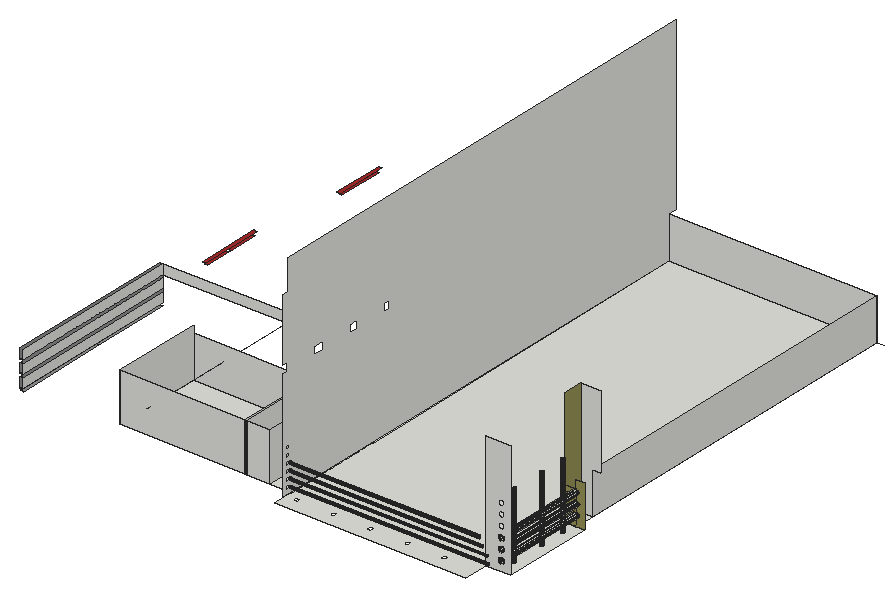
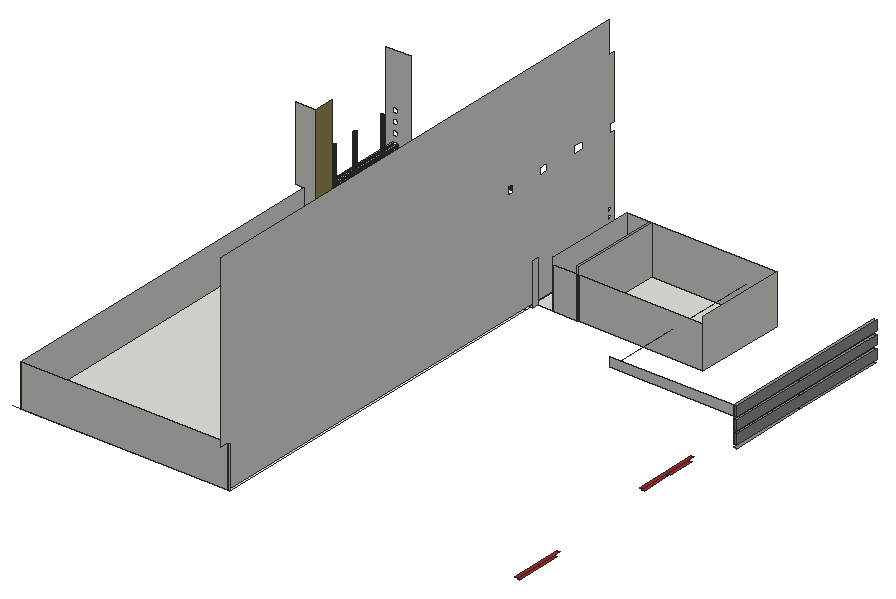
# SketchUp Ruby script. Lengths in inches.
U = 1.inch
M = Sketchup.active_model
def pt(a) = Geom::Point3d.new(a.map { |v| v * U })
def face(e, loops, mat)
  f = e.add_face(loops[0].map { |a| pt(a) })
  loops[1..].each { |l| e.add_face(l.map { |a| pt(a) }).erase! }
  f.material = f.back_material = mat if mat
  f
end
# faces: each face lists its corners as indices into pts; further lists are holes
def faces(e, pts, list, mat = nil) = list.each { |f| face(e, (f[0].is_a?(Array) ? f : [f]).map { |l| l.map { |i| pts[i] } }, mat) }
# xy, xz, yz: faces in a plane at the given z, y or x. An outline is a flat list of corners, or four numbers for a rectangle; further outlines are holes
def ring(l) = l.size == 4 ? [[l[0], l[1]], [l[2], l[1]], [l[2], l[3]], [l[0], l[3]]] : l.each_slice(2).to_a
def flat(e, list, mat, &to3) = list.each { |f| face(e, (f[0].is_a?(Array) ? f : [f]).map { |l| ring(l).map { |u, v| to3.(u, v) } }, mat) }
def xy(e, z, list, mat = nil) = flat(e, list, mat) { |x, y| [x, y, z] }
def xz(e, y, list, mat = nil) = flat(e, list, mat) { |x, z| [x, y, z] }
def yz(e, x, list, mat = nil) = flat(e, list, mat) { |y, z| [x, y, z] }
def lines(e, pts, list) = list.each { |a, b| e.add_line(pt(pts[a]), pt(pts[b])) }
# prism: a flat outline (further loops are holes) pulled along v
def prism(e, loops, v, mat = nil)
  f = face(e, loops, mat); d = Geom::Vector3d.new(v.map { |x| x * U })
  f.pushpull(f.normal.samedirection?(d) ? d.length : -d.length)
end
def box(e, o, s, mat = nil) = prism(e, [[o, [o[0] + s[0], o[1], o[2]], [o[0] + s[0], o[1] + s[1], o[2]], [o[0], o[1] + s[1], o[2]]]], [0, 0, s[2]], mat)
def at(x, y, z, deg = 0) = Geom::Transformation.translation(pt([x, y, z])) * Geom::Transformation.rotation(ORIGIN, Z_AXIS, deg.degrees)
def axes(o, x, y, z) = Geom::Transformation.new([*x, 0, *y, 0, *z, 0, *pt(o).to_a, 1])
def part(name) = M.definitions.add(name)
# library, detail: a bought-in or finely detailed component or shape, given as its bounding box
def library(name, o, s) = part(name).tap { |d| box(d.entities, o, s) }
def detail(e, o, s) = box(e.add_group.entities, o, s)
def put(e, d, t, mat = nil) = e.add_instance(d, t).tap { |i| i.material = mat if mat }
def group(e, t, mat = nil) = e.add_group.tap { |g| g.transformation = t; g.material = mat if mat }.entities
root = M.entities
M.materials.add("[0018_Brown]").color = [165, 42, 42]
M.materials.add("[0057_DarkKhaki]").color = [150, 145, 85]
M.materials.add("[0137_Black]").color = [71, 71, 71]
M.materials.add("[Color M05]").color = [145, 145, 145]
xy(root,378.28,[[8.875,19,11.875,116.75],[8.875,116.75,11.875,199.5]],"[Color M05]")
xy(root,379.4,[[8.875,431.78,11.875,479.72]],"[0018_Brown]")
xy(root,379.43,[[[286.99,1.0625,484.5625,1.0625,484.5625,26.4375,510.6875,26.4375,510.6875,122.75,490.125,122.75,490.125,143.77,501.6875,143.77,501.6875,511.875,286.99,511.875],[412.39,12.9375,411.69,13.03,411.04,13.3,410.49,13.73,410.06,14.28,409.79,14.93,409.7,15.625,409.79,16.32,410.06,16.97,410.49,17.53,411.04,17.95,411.69,18.22,412.39,18.3125,413.08,18.22,413.73,17.95,414.29,17.53,414.72,16.97,414.98,16.32,415.07,15.625,414.98,14.93,414.71,14.28,414.29,13.72,413.73,13.3,413.08,13.03],[450.64,12.9375,449.94,13.03,449.29,13.3,448.74,13.73,448.31,14.28,448.04,14.93,447.95,15.625,448.04,16.32,448.31,16.97,448.74,17.53,449.29,17.95,449.94,18.22,450.64,18.3125,451.33,18.22,451.98,17.95,452.54,17.53,452.97,16.97,453.23,16.32,453.32,15.625,453.23,14.93,452.96,14.28,452.54,13.72,451.98,13.3,451.33,13.03],[297.64,12.9375,296.94,13.03,296.29,13.3,295.74,13.73,295.31,14.28,295.04,14.93,294.95,15.625,295.04,16.32,295.31,16.97,295.74,17.53,296.29,17.95,296.94,18.22,297.64,18.3125,298.33,18.22,298.98,17.95,299.54,17.53,299.97,16.97,300.23,16.32,300.32,15.625,300.23,14.93,299.96,14.28,299.54,13.72,298.98,13.3,298.33,13.03],[335.89,12.9375,335.19,13.03,334.54,13.3,333.99,13.73,333.56,14.28,333.29,14.93,333.2,15.625,333.29,16.32,333.56,16.97,333.99,17.53,334.54,17.95,335.19,18.22,335.89,18.3125,336.58,18.22,337.23,17.95,337.79,17.53,338.22,16.97,338.48,16.32,338.57,15.625,338.48,14.93,338.21,14.28,337.79,13.72,337.23,13.3,336.58,13.03],[374.14,12.9375,373.44,13.03,372.79,13.3,372.24,13.73,371.81,14.28,371.54,14.93,371.45,15.625,371.54,16.32,371.81,16.97,372.24,17.53,372.79,17.95,373.44,18.22,374.14,18.3125,374.83,18.22,375.48,17.95,376.04,17.53,376.47,16.97,376.73,16.32,376.82,15.625,376.73,14.93,376.46,14.28,376.04,13.72,375.48,13.3,374.83,13.03],[499.41,79.41,499.04,79.46,498.6875,79.61,498.39,79.84,498.16,80.13,498.02,80.48,497.97,80.85,498.02,81.22,498.16,81.57,498.39,81.87,498.6875,82.1,499.04,82.24,499.41,82.29,499.78,82.24,500.125,82.1,500.42,81.87,500.65,81.57,500.8,81.22,500.85,80.85,500.8,80.48,500.65,80.13,500.42,79.84,500.125,79.61,499.78,79.46],[499.41,107.04,499.04,107.09,498.6875,107.23,498.39,107.46,498.16,107.76,498.02,108.11,497.97,108.48,498.02,108.85,498.16,109.2,498.39,109.49,498.6875,109.72,499.04,109.87,499.41,109.91,499.78,109.87,500.125,109.72,500.42,109.49,500.65,109.2,500.8,108.85,500.85,108.48,500.8,108.11,500.65,107.76,500.42,107.46,500.125,107.23,499.78,107.09],[499.41,44.29,499.04,44.34,498.6875,44.48,498.39,44.71,498.16,45.01,498.02,45.36,497.97,45.73,498.02,46.1,498.16,46.45,498.39,46.74,498.6875,46.97,499.04,47.12,499.41,47.16,499.78,47.12,500.125,46.97,500.42,46.74,500.65,46.45,500.8,46.1,500.85,45.73,500.8,45.36,500.65,45.01,500.42,44.71,500.125,44.48,499.78,44.34]],[286.17,18.1875,286.99,22.0625],[284.05,22.0625,284.05,22.07,284.41,22.0625],[284.41,22.0625,284.05,22.07,284.05,116.75,284.41,116.75],[284.41,22.0625,284.41,116.75,285.29,116.75],
  [284.41,22.0625,285.29,116.75,285.29,22.0625],[285.29,22.0625,286.17,116.75],[286.17,22.0625,286.99,116.75],[284.05,22.07,264.04,22.25,264.92,116.9375,281.04,116.79,281.04,116.75,284.05,116.75],[264.04,22.25,239.85,22.47,240.73,117.16,264.92,116.9375],
  [239.85,22.47,237.79,22.49,238.67,117.18,240.73,117.16],[237.79,22.49,107.8,23.69,108.67,118.38,238.67,117.18],[281.04,116.75,281.04,116.79,284.05,116.76,284.05,116.75],[284.05,116.75,284.05,116.76,285.29,116.75],[285.29,116.75,284.05,116.76,284.05,122.75,285.29,122.75],
  [285.29,116.75,286.17,122.75],[286.17,116.75,286.99,122.75],[284.05,116.76,281.04,116.79,281.04,122.75,284.05,122.75],[284.05,122.75,286.17,128.75],[286.17,122.75,286.99,128.75],
  [490.125,122.75,501.6875,143.77],[284.05,128.75,286.17,511.875],[286.17,128.75,286.99,511.875]])
xy(root,381.32,[[8.875,18.1875,11.875,199.5]])
xy(root,382.4,[[8.875,428.78,11.875,482.72]],"[0018_Brown]")
xy(root,391.28,[[8.875,257.47,11.875,284.61],[8.875,287.91,11.875,318.35]],"[0018_Brown]")
xy(root,391.4,[[8.875,18.1875,11.875,116.75],[8.875,116.75,11.875,199.5]],"[Color M05]")
xy(root,394.28,[[8.875,254.47,11.875,321.35]],"[0018_Brown]")
xy(root,394.44,[[8.875,18.1875,11.875,199.5]])
xy(root,404.53,[[8.875,18.1875,11.875,116.75],[8.875,116.75,11.875,199.5]],"[Color M05]")
xy(root,407.57,[[8.875,18.1875,11.875,199.5]])
xz(root,26.4375,[[[484.5625,379.43,510.6875,499.43],[501.3,386.68,502.06,386.78,502.77,387.07,503.375,387.54,503.84,388.15,504.13,388.85,504.23,389.62,504.13,390.375,503.84,391.08,503.375,391.69,502.77,392.16,502.06,392.45,501.3,392.55,500.54,392.45,499.83,392.16,499.22,391.69,498.75,391.08,498.46,390.375,498.36,389.62,498.46,388.85,498.75,388.15,499.22,387.54,499.83,387.07,500.54,386.78],[501.3,397.43,502.06,397.53,502.77,397.82,503.375,398.29,503.84,398.9,504.13,399.6,504.23,400.37,504.13,401.125,503.84,401.83,503.375,402.44,502.77,402.91,502.06,403.2,501.3,403.3,500.54,403.2,499.83,402.91,499.22,402.44,498.75,401.83,498.46,401.125,498.36,400.37,498.46,399.6,498.75,398.9,499.22,398.29,499.83,397.82,500.54,397.53],[501.3,408.18,502.06,408.28,502.77,408.57,503.375,409.04,503.84,409.65,504.13,410.35,504.23,411.12,504.13,411.875,503.84,412.58,503.375,413.19,502.77,413.66,502.06,413.95,501.3,414.05,500.54,413.95,499.83,413.66,499.22,413.19,498.75,412.58,498.46,411.875,498.36,411.12,498.46,410.35,498.75,409.65,499.22,409.04,499.83,408.57,500.54,408.28],[501.3,418.93,502.06,419.03,502.77,419.32,503.375,419.79,503.84,420.4,504.13,421.1,504.23,421.87,504.13,422.625,503.84,423.33,503.375,423.94,502.77,424.41,502.06,424.7,501.3,424.8,500.54,424.7,499.83,424.41,499.22,423.94,498.75,423.33,498.46,422.625,498.36,421.87,498.46,421.1,498.75,420.4,499.22,419.79,499.83,419.32,500.54,419.03],[501.3,429.68,502.06,429.78,502.77,430.07,503.375,430.54,503.84,431.15,504.13,431.85,504.23,432.62,504.13,433.375,503.84,434.08,503.375,434.69,502.77,435.16,502.06,435.45,501.3,435.55,500.54,435.45,499.83,435.16,499.22,434.69,498.75,434.08,498.46,433.375,498.36,432.62,498.46,431.85,498.75,431.15,499.22,430.54,499.83,430.07,500.54,429.78],[501.3,440.43,502.06,440.53,502.77,440.82,503.375,441.29,503.84,441.9,504.13,442.6,504.23,443.37,504.13,444.125,503.84,444.83,503.375,445.44,502.77,445.91,502.06,446.2,501.3,446.3,500.54,446.2,499.83,445.91,499.22,445.44,498.75,444.83,498.46,444.125,498.36,443.37,498.46,442.6,498.75,441.9,499.22,441.29,499.83,440.82,500.54,440.53]]])
xz(root,122.75,[[501.3,408.18,500.91,408.23,501.6875,408.23],[500.91,408.23,500.54,408.28,499.83,408.57,499.22,409.04,498.75,409.65,498.46,410.35,498.36,411.12,498.46,411.875,498.75,412.58,499.22,413.19,499.83,413.66,500.54,413.95,500.91,414,501.6875,414,501.6875,408.23],[501.6875,408.23,501.6875,414,502.06,413.95,502.77,413.66,503.375,413.19,503.84,412.58,504.13,411.875,504.23,411.12,504.13,410.35,503.84,409.65,503.375,409.04,502.77,408.57,502.06,408.28]])
xz(root,122.75,[[490.125,379.43,501.6875,379.43,501.6875,408.23,501.3,408.18,500.91,408.23,490.125,408.23],[501.6875,379.43,510.6875,379.43,510.6875,423,501.6875,423,501.6875,414,502.06,413.95,502.77,413.66,503.375,413.19,503.84,412.58,504.13,411.875,504.23,411.12,504.13,410.35,503.84,409.65,503.375,409.04,502.77,408.57,502.06,408.28,501.6875,408.23],[490.125,408.23,500.91,408.23,500.54,408.28,499.83,408.57,499.22,409.04,498.75,409.65,498.46,410.35,498.36,411.12,498.46,411.875,498.75,412.58,499.22,413.19,499.83,413.66,500.54,413.95,500.91,414,490.125,414]],"[0057_DarkKhaki]")
xz(root,123.3125,[[501.3,386.68,500.54,386.78,499.83,387.07,499.22,387.54,498.75,388.15,498.46,388.85,498.36,389.62,498.46,390.375,498.75,391.08,499.22,391.69,499.83,392.16,500.54,392.45,501.3,392.55,502.06,392.45,502.77,392.16,503.375,391.69,503.84,391.08,504.13,390.375,504.23,389.62,504.13,388.85,503.84,388.15,503.375,387.54,502.77,387.07,502.06,386.78]])
xz(root,127.4375,[[501.3,397.43,500.54,397.53,499.83,397.82,499.22,398.29,498.75,398.9,498.46,399.6,498.36,400.37,498.46,401.125,498.75,401.83,499.22,402.44,499.83,402.91,500.54,403.2,501.3,403.3,502.06,403.2,502.77,402.91,503.375,402.44,503.84,401.83,504.13,401.125,504.23,400.37,504.13,399.6,503.84,398.9,503.375,398.29,502.77,397.82,502.06,397.53]])
xz(root,143.77,[[490.125,379.43,490.125,499.43,510.6875,499.43,510.6875,423,501.6875,423,501.6875,379.43]])
xz(root,199.5,[[11.875,407.57,139.9375,417.65]])
xz(root,199.5,[[8.875,381.32,11.875,391.4],[8.875,394.44,11.875,404.53],[8.875,407.57,11.875,417.65]],"[Color M05]")
xz(root,511.875,[[284.05,379.43,286.17,423],[286.17,379.43,501.6875,423]])
yz(root,8.875,[[18.1875,381.32,199.5,391.4],[18.1875,394.44,199.5,404.53],[18.1875,407.57,199.5,417.65]],"[Color M05]")
yz(root,11.875,[[19,381.32,199.5,381.32,199.5,391.4,18.1875,391.4,18.1875,381.65,19,381.65],[18.1875,394.44,199.5,404.53],[18.1875,407.57,199.5,417.65]])
yz(root,11.875,[[18.1875,391.4,199.5,394.44],[18.1875,404.53,199.5,407.57]],"[Color M05]")
yz(root,281.04,[[116.75,379.43,122.75,423]])
yz(root,286.17,[[[12.1875,379.43,511.875,379.43,511.875,423,520.875,423,520.875,599.125,18.1875,599.125,18.1875,567.22,12.1875,567.22,12.1875,501.97,16.9375,501.97,16.9375,493.97,12.1875,493.97],[51.75,493.97,63.75,501.97],[98.5625,493.97,108.4375,501.97],[143.25,493.97,149.48,501.97],[18.04,383.86,17.46,383.94,16.92,384.16,16.45,384.52,16.1,384.99,15.87,385.53,15.79,386.11,15.87,386.7,16.1,387.24,16.45,387.7,16.92,388.0625,17.46,388.29,18.04,388.36,18.63,388.29,19.17,388.0625,19.64,387.7,19.99,387.24,20.22,386.7,20.29,386.11,20.22,385.53,19.99,384.99,19.64,384.52,19.17,384.16,18.63,383.94],[18.04,391.36,17.46,391.44,16.92,391.66,16.45,392.02,16.1,392.49,15.87,393.03,15.79,393.61,15.87,394.2,16.1,394.74,16.45,395.2,16.92,395.5625,17.46,395.79,18.04,395.86,18.63,395.79,19.17,395.5625,19.64,395.2,19.99,394.74,20.22,394.2,20.29,393.61,20.22,393.03,19.99,392.49,19.64,392.02,19.17,391.66,18.63,391.44],[18.04,398.86,17.46,398.94,16.92,399.16,16.45,399.52,16.1,399.99,15.87,400.53,15.79,401.11,15.87,401.7,16.1,402.24,16.45,402.7,16.92,403.0625,17.46,403.29,18.04,403.36,18.63,403.29,19.17,403.0625,19.64,402.7,19.99,402.24,20.22,401.7,20.29,401.11,20.22,400.53,19.99,399.99,19.64,399.52,19.17,399.16,18.63,398.94],[18.04,406.36,17.46,406.44,16.92,406.66,16.45,407.02,16.1,407.49,15.87,408.03,15.79,408.61,15.87,409.2,16.1,409.74,16.45,410.2,16.92,410.5625,17.46,410.79,18.04,410.86,18.63,410.79,19.17,410.5625,19.64,410.2,19.99,409.74,20.22,409.2,20.29,408.61,20.22,408.03,19.99,407.49,19.64,407.02,19.17,406.66,18.63,406.44],[18.04,413.86,17.46,413.94,16.92,414.16,16.45,414.52,16.1,414.99,15.87,415.53,15.79,416.11,15.87,416.7,16.1,417.24,16.45,417.7,16.92,418.0625,17.46,418.29,18.04,418.36,18.63,418.29,19.17,418.0625,19.64,417.7,19.99,417.24,20.22,416.7,20.29,416.11,20.22,415.53,19.99,414.99,19.64,414.52,19.17,414.16,18.63,413.94],[18.04,421.36,17.46,421.44,16.92,421.66,16.45,422.02,16.1,422.49,15.87,423.03,15.79,423.61,15.87,424.2,16.1,424.74,16.45,425.2,16.92,425.5625,17.46,425.79,18.04,425.86,18.63,425.79,19.17,425.5625,19.64,425.2,19.99,424.74,20.22,424.2,20.29,423.61,20.22,423.03,19.99,422.49,19.64,422.02,19.17,421.66,18.63,421.44]]])
yz(root,490.125,[[122.75,379.43,143.77,499.43]],"[0057_DarkKhaki]")
yz(root,501.6875,[[143.77,379.43,511.875,423]])
p = [[264.04,22.25,429.99],[239.85,22.47,429.99],[239.85,22.47,379.43],[264.04,22.25,379.43],[264.91,116.51,429.99],[264.91,116.75,429.99],
  [264.92,116.9375,429.99],[264.92,116.9375,423],[264.92,116.9375,379.43],[107.8,23.69,379.43],[237.79,22.49,379.43],[237.79,22.49,429.99],
  [107.8,23.69,429.99],[238.66,116.75,429.99],[238.67,117.18,429.99],[238.67,117.18,423],[238.67,117.18,379.43],[240.73,116.73,429.99],
  [240.73,116.75,429.99],[240.73,117.16,429.99],[240.73,117.16,423],[240.73,117.16,379.43],[108.66,116.75,429.99],[108.67,118.38,429.99],
  [108.67,118.38,423],[108.67,118.38,379.43],[498.6875,44.48,379.43],[499.04,44.34,379.43],[499.04,44.34,448.18],[498.6875,44.48,448.18],
  [499.41,44.29,379.43],[499.41,44.29,448.18],[499.78,44.34,379.43],[499.78,44.34,448.18],[500.125,44.48,379.43],[500.125,44.48,448.18],
  [498.39,44.71,379.43],[498.39,44.71,448.18],[500.42,44.71,379.43],[500.42,44.71,448.18],[498.16,45.01,379.43],[498.16,45.01,448.18],
  [500.65,45.01,379.43],[500.65,45.01,448.18],[498.02,45.36,379.43],[498.02,45.36,448.18],[500.8,45.36,379.43],[500.8,45.36,448.18],
  [497.97,45.73,379.43],[497.97,45.73,448.18],[500.85,45.73,379.43],[500.85,45.73,448.18],[498.02,46.1,379.43],[498.02,46.1,448.18],
  [500.8,46.1,379.43],[500.8,46.1,448.18],[498.16,46.45,379.43],[498.16,46.45,448.18],[500.65,46.45,379.43],[500.65,46.45,448.18],
  [498.39,46.74,379.43],[498.39,46.74,448.18],[500.42,46.74,379.43],[500.42,46.74,448.18],[498.6875,46.97,379.43],[498.6875,46.97,448.18],
  [500.125,46.97,379.43],[500.125,46.97,448.18],[499.04,47.12,379.43],[499.04,47.12,448.18],[499.78,47.12,379.43],[499.78,47.12,448.18],
  [499.41,47.16,379.43],[499.41,47.16,448.18],[499.04,79.46,379.43],[499.41,79.41,379.43],[499.41,79.41,448.18],[499.04,79.46,448.18],
  [499.78,79.46,379.43],[499.78,79.46,448.18],[498.6875,79.61,379.43],[498.6875,79.61,448.18],[500.125,79.61,379.43],[500.125,79.61,448.18],
  [498.39,79.84,379.43],[498.39,79.84,448.18],[500.42,79.84,379.43],[500.42,79.84,448.18],[498.16,80.13,379.43],[498.16,80.13,448.18],
  [500.65,80.13,379.43],[500.65,80.13,448.18],[498.02,80.48,379.43],[498.02,80.48,448.18],[500.8,80.48,379.43],[500.8,80.48,448.18],
  [497.97,80.85,379.43],[497.97,80.85,448.18],[500.85,80.85,379.43],[500.85,80.85,448.18],[498.02,81.22,379.43],[498.02,81.22,448.18],
  [500.8,81.22,379.43],[500.8,81.22,448.18],[498.16,81.57,379.43],[498.16,81.57,448.18],[500.65,81.57,379.43],[500.65,81.57,448.18],
  [498.39,81.87,379.43],[498.39,81.87,448.18],[500.42,81.87,379.43],[500.42,81.87,448.18],[498.6875,82.1,379.43],[498.6875,82.1,448.18],
  [500.125,82.1,379.43],[500.125,82.1,448.18],[499.04,82.24,379.43],[499.04,82.24,448.18],[499.78,82.24,379.43],[499.78,82.24,448.18],
  [499.41,82.29,379.43],[499.41,82.29,448.18],[499.04,107.09,379.43],[499.41,107.04,379.43],[499.41,107.04,448.18],[499.04,107.09,448.18],
  [499.78,107.09,379.43],[499.78,107.09,448.18],[498.6875,107.23,379.43],[498.6875,107.23,448.18],[500.125,107.23,379.43],[500.125,107.23,448.18],
  [498.39,107.46,379.43],[498.39,107.46,448.18],[500.42,107.46,379.43],[500.42,107.46,448.18],[498.16,107.76,379.43],[498.16,107.76,448.18],
  [500.65,107.76,379.43],[500.65,107.76,448.18],[498.02,108.11,379.43],[498.02,108.11,448.18],[500.8,108.11,379.43],[500.8,108.11,448.18],
  [497.97,108.48,379.43],[497.97,108.48,448.18],[500.85,108.48,379.43],[500.85,108.48,448.18],[498.02,108.85,379.43],[498.02,108.85,448.18],
  [500.8,108.85,379.43],[500.8,108.85,448.18],[498.16,109.2,379.43],[498.16,109.2,448.18],[500.65,109.2,379.43],[500.65,109.2,448.18],
  [498.39,109.49,379.43],[498.39,109.49,448.18],[500.42,109.49,379.43],[500.42,109.49,448.18],[498.6875,109.72,379.43],[498.6875,109.72,448.18],
  [500.125,109.72,379.43],[500.125,109.72,448.18],[499.04,109.87,379.43],[499.04,109.87,448.18],[499.78,109.87,379.43],[499.78,109.87,448.18],
  [499.41,109.91,379.43],[499.41,109.91,448.18],[286.17,19.99,384.99],[286.17,20.22,385.53],[492.98,20.22,385.53],[492.98,19.99,384.99],
  [286.17,20.29,386.11],[492.98,20.29,386.11],[286.17,20.22,386.7],[492.98,20.22,386.7],[286.17,19.99,387.24],[492.98,19.99,387.24],
  [501.3,26.4375,386.68],[500.54,26.4375,386.78],[500.54,123.3125,386.78],[501.3,123.3125,386.68],[502.06,26.4375,386.78],[502.06,123.3125,386.78],
  [499.83,26.4375,387.07],[499.83,123.3125,387.07],[502.77,26.4375,387.07],[502.77,123.3125,387.07],[499.22,26.4375,387.54],[499.22,123.3125,387.54],
  [503.375,26.4375,387.54],[503.375,123.3125,387.54],[498.75,26.4375,388.15],[498.75,123.3125,388.15],[503.84,26.4375,388.15],[503.84,123.3125,388.15],
  [498.46,26.4375,388.85],[498.46,123.3125,388.85],[504.13,26.4375,388.85],[504.13,123.3125,388.85],[498.36,26.4375,389.62],[498.36,123.3125,389.62],
  [504.23,26.4375,389.62],[504.23,123.3125,389.62],[498.46,26.4375,390.375],[498.46,123.3125,390.375],[504.13,26.4375,390.375],[504.13,123.3125,390.375],
  [498.75,26.4375,391.08],[498.75,123.3125,391.08],[503.84,26.4375,391.08],[503.84,123.3125,391.08],[499.22,26.4375,391.69],[499.22,123.3125,391.69],
  [503.375,26.4375,391.69],[503.375,123.3125,391.69],[499.83,26.4375,392.16],[499.83,123.3125,392.16],[502.77,26.4375,392.16],[502.77,123.3125,392.16],
  [500.54,26.4375,392.45],[500.54,123.3125,392.45],[502.06,26.4375,392.45],[502.06,123.3125,392.45],[286.17,19.99,392.49],[286.17,20.22,393.03],
  [492.3,20.22,393.03],[492.3,19.99,392.49],[501.3,26.4375,392.55],[501.3,123.3125,392.55],[286.17,20.29,393.61],[492.3,20.29,393.61],
  [286.17,20.22,394.2],[492.3,20.22,394.2],[286.17,19.99,394.74],[492.3,19.99,394.74],[286.17,19.64,395.2],[492.3,19.64,395.2],
  [501.3,26.4375,397.43],[500.54,26.4375,397.53],[500.54,127.4375,397.53],[501.3,127.4375,397.43],[502.06,26.4375,397.53],[502.06,127.4375,397.53],
  [499.83,26.4375,397.82],[499.83,127.4375,397.82],[502.77,26.4375,397.82],[502.77,127.4375,397.82],[499.22,26.4375,398.29],[499.22,127.4375,398.29],
  [503.375,26.4375,398.29],[503.375,127.4375,398.29],[498.75,26.4375,398.9],[498.75,127.4375,398.9],[503.84,26.4375,398.9],[503.84,127.4375,398.9],
  [498.46,26.4375,399.6],[498.46,127.4375,399.6],[504.13,26.4375,399.6],[504.13,127.4375,399.6],[286.17,19.64,399.52],[286.17,19.99,399.99],
  [487.23,19.99,399.99],[487.23,19.64,399.52],[498.36,26.4375,400.37],[498.36,127.4375,400.37],[504.23,26.4375,400.37],[504.23,127.4375,400.37],
  [286.17,20.22,400.53],[487.23,20.22,400.53],[498.46,26.4375,401.125],[498.46,127.4375,401.125],[504.13,26.4375,401.125],[504.13,127.4375,401.125],
  [286.17,20.29,401.11],[487.23,20.29,401.11],[286.17,20.22,401.7],[487.23,20.22,401.7],[498.75,26.4375,401.83],[498.75,127.4375,401.83],
  [503.84,26.4375,401.83],[503.84,127.4375,401.83],[286.17,19.99,402.24],[487.23,19.99,402.24],[499.22,26.4375,402.44],[499.22,127.4375,402.44],
  [503.375,26.4375,402.44],[503.375,127.4375,402.44],[286.17,19.64,402.7],[487.23,19.64,402.7],[499.83,26.4375,402.91],[499.83,127.4375,402.91],
  [502.77,26.4375,402.91],[502.77,127.4375,402.91],[500.54,26.4375,403.2],[500.54,127.4375,403.2],[502.06,26.4375,403.2],[502.06,127.4375,403.2],
  [501.3,26.4375,403.3],[501.3,127.4375,403.3],[286.17,19.64,407.02],[286.17,19.99,407.49],[484.11,19.99,407.49],[484.11,19.64,407.02],
  [286.17,20.22,408.03],[484.11,20.22,408.03],[286.17,20.29,408.61],[484.11,20.29,408.61],[501.3,26.4375,408.18],[500.54,26.4375,408.28],
  [500.54,122.75,408.28],[500.91,122.75,408.23],[501.3,122.75,408.18],[502.06,26.4375,408.28],[501.6875,122.75,408.23],[502.06,122.75,408.28],
  [499.83,26.4375,408.57],[499.83,122.75,408.57],[502.77,26.4375,408.57],[502.77,122.75,408.57],[286.17,20.22,409.2],[484.11,20.22,409.2],
  [499.22,26.4375,409.04],[499.22,122.75,409.04],[503.375,26.4375,409.04],[503.375,122.75,409.04],[498.75,26.4375,409.65],[498.75,122.75,409.65],
  [503.84,26.4375,409.65],[503.84,122.75,409.65],[286.17,19.99,409.74],[484.11,19.99,409.74],[498.46,26.4375,410.35],[498.46,122.75,410.35],
  [504.13,26.4375,410.35],[504.13,122.75,410.35],[286.17,19.64,410.2],[484.11,19.64,410.2],[498.36,26.4375,411.12],[498.36,122.75,411.12],
  [504.23,26.4375,411.12],[504.23,122.75,411.12],[498.46,26.4375,411.875],[498.46,122.75,411.875],[504.13,26.4375,411.875],[504.13,122.75,411.875],
  [498.75,26.4375,412.58],[498.75,122.75,412.58],[503.84,26.4375,412.58],[503.84,122.75,412.58],[499.22,26.4375,413.19],[499.22,122.75,413.19],
  [503.375,26.4375,413.19],[503.375,122.75,413.19],[501.6875,511.875,379.43],[509.9375,511.875,379.43],[139.9375,18.1875,407.57],[139.9375,199.5,407.57]]
faces(root,p,[[0,1,2,3],[0,4,5,6,7,8,3],[9,10,11,12],[10,2,1,11],[11,13,14,15,16,10],[1,17,18,19,20,21,2],[12,22,23,24,25,9],[26,27,28,29],
  [27,30,31,28],[30,32,33,31],[32,34,35,33],[36,26,29,37],[34,38,39,35],[40,36,37,41],[38,42,43,39],[44,40,41,45],
  [42,46,47,43],[48,44,45,49],[46,50,51,47],[52,48,49,53],[50,54,55,51],[56,52,53,57],[54,58,59,55],[60,56,57,61],
  [58,62,63,59],[64,60,61,65],[62,66,67,63],[68,64,65,69],[66,70,71,67],[72,68,69,73],[70,72,73,71],[74,75,76,77],
  [75,78,79,76],[80,74,77,81],[78,82,83,79],[84,80,81,85],[82,86,87,83],[88,84,85,89],[86,90,91,87],[92,88,89,93],
  [90,94,95,91],[96,92,93,97],[94,98,99,95],[100,96,97,101],[98,102,103,99],[104,100,101,105],[102,106,107,103],[108,104,105,109],
  [106,110,111,107],[112,108,109,113],[110,114,115,111],[116,112,113,117],[114,118,119,115],[120,116,117,121],[118,120,121,119],[122,123,124,125],
  [123,126,127,124],[128,122,125,129],[126,130,131,127],[132,128,129,133],[130,134,135,131],[136,132,133,137],[134,138,139,135],[140,136,137,141],
  [138,142,143,139],[144,140,141,145],[142,146,147,143],[148,144,145,149],[146,150,151,147],[152,148,149,153],[150,154,155,151],[156,152,153,157],
  [154,158,159,155],[160,156,157,161],[158,162,163,159],[164,160,161,165],[162,166,167,163],[168,164,165,169],[166,168,169,167],[8,21,20,7],
  [24,15,16,25],[15,20,21,16],[180,181,182,183],[184,180,183,185],[181,186,187,182],[188,184,185,189],[186,190,191,187],[192,188,189,193],
  [190,194,195,191],[196,192,193,197],[194,198,199,195],[200,196,197,201],[198,202,203,199],[204,200,201,205],[202,206,207,203],[208,204,205,209],
  [206,210,211,207],[212,208,209,213],[210,214,215,211],[216,212,213,217],[214,218,219,215],[220,216,217,221],[218,222,223,219],[224,220,221,225],
  [222,230,231,223],[230,224,225,231],[240,241,242,243],[244,240,243,245],[241,246,247,242],[248,244,245,249],[246,250,251,247],[252,248,249,253],
  [250,254,255,251],[256,252,253,257],[254,258,259,255],[260,256,257,261],[258,266,267,259],[268,260,261,269],[266,272,273,267],[274,268,269,275],
  [272,280,281,273],[282,274,275,283],[280,286,287,281],[288,282,283,289],[286,292,293,287],[294,288,289,295],[292,296,297,293],[298,294,295,299],
  [296,300,301,297],[300,298,299,301],[310,311,312,313,314],[315,310,314,316,317],[311,318,319,312],[320,315,317,321],[318,324,325,319],[326,320,321,327],
  [324,328,329,325],[330,326,327,331],[328,334,335,329],[336,330,331,337],[334,340,341,335],[342,336,337,343],[340,344,345,341],[346,342,343,347],
  [344,348,349,345],[350,346,347,351],[348,352,353,349],[354,350,351,355]])
faces(root,p,[[170,171,172,173],[171,174,175,172],[174,176,177,175],[176,178,179,177],[226,227,228,229],[227,232,233,228],[232,234,235,233],[234,236,237,235],
  [236,238,239,237],[262,263,264,265],[263,270,271,264],[270,276,277,271],[276,278,279,277],[278,284,285,279],[284,290,291,285],[302,303,304,305],
  [303,306,307,304],[306,308,309,307],[308,322,323,309],[322,332,333,323],[332,338,339,333]],"[0137_Black]")
lines(root,p,[[356,357],[358,359]])
